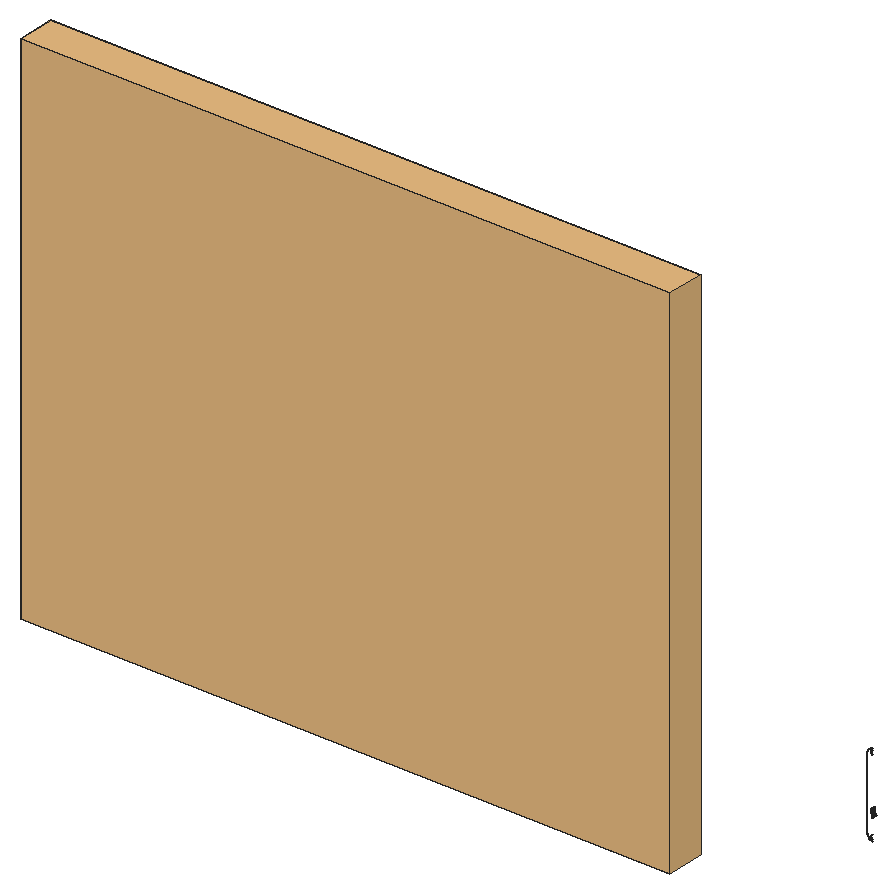
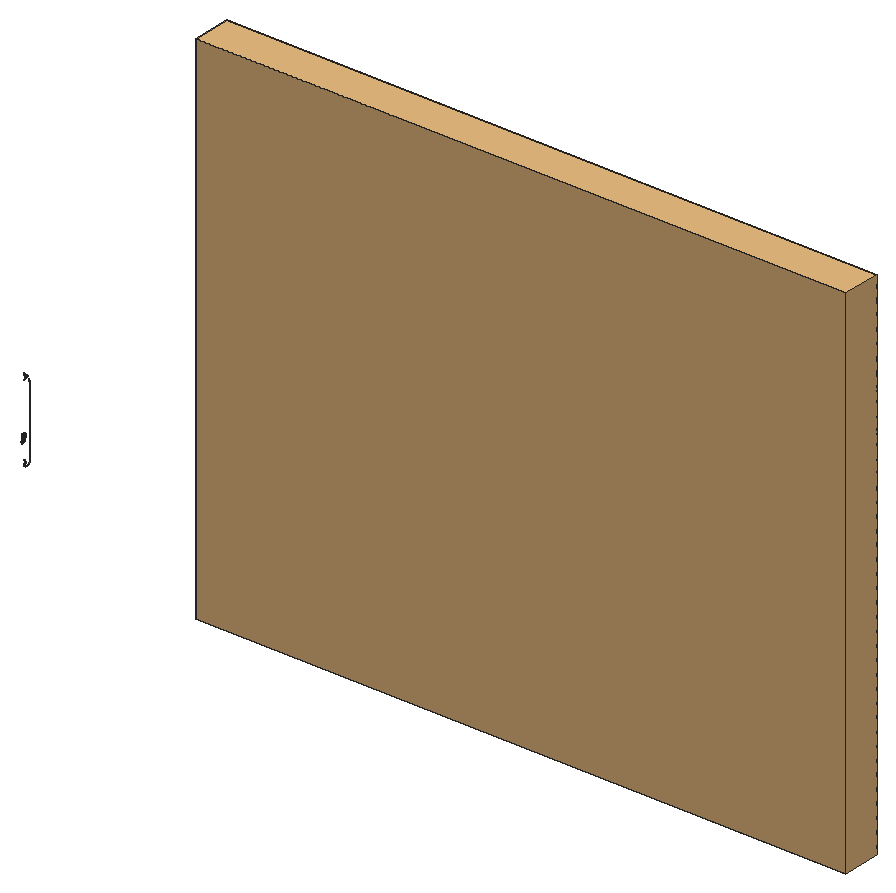
# SketchUp Ruby script. Lengths in inches.
U = 1.inch
M = Sketchup.active_model
def pt(a) = Geom::Point3d.new(a.map { |v| v * U })
def face(e, loops, mat)
  f = e.add_face(loops[0].map { |a| pt(a) })
  loops[1..].each { |l| e.add_face(l.map { |a| pt(a) }).erase! }
  f.material = f.back_material = mat if mat
  f
end
# faces: each face lists its corners as indices into pts; further lists are holes
def faces(e, pts, list, mat = nil) = list.each { |f| face(e, (f[0].is_a?(Array) ? f : [f]).map { |l| l.map { |i| pts[i] } }, mat) }
# xy, xz, yz: faces in a plane at the given z, y or x. An outline is a flat list of corners, or four numbers for a rectangle; further outlines are holes
def ring(l) = l.size == 4 ? [[l[0], l[1]], [l[2], l[1]], [l[2], l[3]], [l[0], l[3]]] : l.each_slice(2).to_a
def flat(e, list, mat, &to3) = list.each { |f| face(e, (f[0].is_a?(Array) ? f : [f]).map { |l| ring(l).map { |u, v| to3.(u, v) } }, mat) }
def xy(e, z, list, mat = nil) = flat(e, list, mat) { |x, y| [x, y, z] }
def xz(e, y, list, mat = nil) = flat(e, list, mat) { |x, z| [x, y, z] }
def yz(e, x, list, mat = nil) = flat(e, list, mat) { |y, z| [x, y, z] }
def lines(e, pts, list) = list.each { |a, b| e.add_line(pt(pts[a]), pt(pts[b])) }
# prism: a flat outline (further loops are holes) pulled along v
def prism(e, loops, v, mat = nil)
  f = face(e, loops, mat); d = Geom::Vector3d.new(v.map { |x| x * U })
  f.pushpull(f.normal.samedirection?(d) ? d.length : -d.length)
end
def box(e, o, s, mat = nil) = prism(e, [[o, [o[0] + s[0], o[1], o[2]], [o[0] + s[0], o[1] + s[1], o[2]], [o[0], o[1] + s[1], o[2]]]], [0, 0, s[2]], mat)
def at(x, y, z, deg = 0) = Geom::Transformation.translation(pt([x, y, z])) * Geom::Transformation.rotation(ORIGIN, Z_AXIS, deg.degrees)
def axes(o, x, y, z) = Geom::Transformation.new([*x, 0, *y, 0, *z, 0, *pt(o).to_a, 1])
def part(name) = M.definitions.add(name)
# library, detail: a bought-in or finely detailed component or shape, given as its bounding box
def library(name, o, s) = part(name).tap { |d| box(d.entities, o, s) }
def detail(e, o, s) = box(e.add_group.entities, o, s)
def put(e, d, t, mat = nil) = e.add_instance(d, t).tap { |i| i.material = mat if mat }
def group(e, t, mat = nil) = e.add_group.tap { |g| g.transformation = t; g.material = mat if mat }.entities
root = M.entities
M.materials.add("Material \#1").color = [140, 140, 140]
c1 = library("Multi-panel window",[0,0,0],[5.02,84.63,60])
xz(root,196.7,[[109.188,40.003,109.081,40.059,109.128,40.018],[109.188,40.003,109.128,40.018,109.157,40.007],[109.128,40.018,109.081,40.059,109.102,40.036],[109.295,40.059,108.945,40.647,109.046,40.46],[109.295,40.059,109.019,40.535,108.945,40.647],
  [109.295,40.059,109.053,40.498,109.019,40.535],[109.295,40.059,109.046,40.46,109.048,40.455],[109.295,40.059,109.048,40.455,109.05,40.45],[109.295,40.059,109.05,40.45,109.051,40.444],[109.081,40.059,109.051,40.438,109.054,40.118],
  [109.081,40.059,109.051,40.444,109.051,40.438],[109.081,40.059,109.295,40.059,109.051,40.444],[109.295,40.059,109.093,40.471,109.053,40.498],[109.081,40.059,109.054,40.118,109.065,40.087],[109.295,40.059,109.138,40.453,109.093,40.471],
  [109.054,40.118,109.051,40.438,109.051,40.152],[109.046,40.46,108.945,40.647,109.042,40.466],[109.042,40.466,108.945,40.647,109.039,40.47],[109.039,40.47,108.945,40.647,108.991,40.523],[109.039,40.47,108.991,40.523,109.034,40.475],
  [109.034,40.475,108.991,40.523,109.011,40.497],[108.991,40.523,108.945,40.647,108.961,40.581],[108.991,40.523,108.961,40.581,108.975,40.551],[109.019,40.535,108.993,40.579,108.945,40.647],[108.993,40.579,108.977,40.628,108.945,40.647],
  [108.961,40.581,108.945,40.647,108.951,40.613],[108.977,40.628,108.971,40.682,108.945,40.647],[108.945,40.647,108.949,40.743,108.943,40.682],[108.945,40.647,108.971,40.682,108.977,40.736],[108.945,40.647,108.977,40.736,108.996,40.849],
  [108.945,40.647,108.996,40.849,108.949,40.743],[108.977,40.736,108.993,40.786,108.996,40.849],[108.949,40.743,108.996,40.849,108.967,40.8],[108.993,40.786,109.019,40.829,108.996,40.849],[109.019,40.829,109.053,40.866,108.996,40.849],
  [108.996,40.849,109.053,40.866,109.093,40.894],[108.996,40.849,109.08,40.922,109.035,40.89],[108.996,40.849,109.093,40.894,109.188,40.949],[108.996,40.849,109.188,40.949,109.08,40.922],[109.093,40.894,109.138,40.912,109.188,40.949],
  [109.138,40.912,109.188,40.918,109.188,40.949],[109.08,40.922,109.188,40.949,109.132,40.942]],"Material \#1")
xz(root,196.734,[[109.188,37.641,109.188,37.652,109.074,37.652],[109.074,37.652,109.076,37.663,108.968,37.684],[109.074,37.652,109.188,37.652,109.076,37.663],[109.076,37.663,108.972,37.695,108.968,37.684],[108.968,37.684,108.972,37.695,108.869,37.734],
  [108.972,37.695,108.875,37.745,108.869,37.734],[108.869,37.734,108.875,37.745,108.781,37.802],[108.875,37.745,108.788,37.811,108.781,37.802],[108.781,37.802,108.788,37.811,108.705,37.885],[108.788,37.811,108.713,37.893,108.705,37.885],
  [109.188,37.824,109.188,37.836,109.151,37.828],[109.151,37.828,109.152,37.84,109.115,37.839],[109.151,37.828,109.188,37.836,109.152,37.84],[109.115,37.839,109.119,37.85,109.082,37.855],[109.115,37.839,109.152,37.84,109.119,37.85],
  [109.119,37.85,109.088,37.866,109.082,37.855],[109.082,37.855,109.088,37.866,109.053,37.878],[109.088,37.866,109.06,37.887,109.053,37.878],[109.053,37.878,109.06,37.887,109.028,37.905],[108.705,37.885,108.713,37.893,108.646,37.975],
  [109.06,37.887,109.036,37.913,109.028,37.905],[108.713,37.893,108.655,37.981,108.646,37.975],[109.028,37.905,109.036,37.913,109.007,37.937],[109.036,37.913,109.016,37.943,109.007,37.937],[109.007,37.937,109.016,37.943,108.991,37.973],
  [109.016,37.943,109.002,37.977,108.991,37.973],[108.991,37.973,109.002,37.977,108.982,38.011],[108.646,37.975,108.655,37.981,108.596,38.088],[109.002,37.977,108.992,38.014,108.982,38.011],[108.655,37.981,108.606,38.092,108.596,38.088],
  [108.982,38.011,108.992,38.014,108.978,38.048],[108.992,38.014,108.989,38.048,108.978,38.048],[108.978,38.048,108.989,38.048,108.982,38.093],[108.989,38.048,108.992,38.091,108.982,38.093],[108.596,38.088,108.606,38.092,108.567,38.204],
  [108.992,38.091,108.991,38.132,108.982,38.093],[108.992,38.091,109.002,38.128,108.991,38.132],[108.606,38.092,108.577,38.206,108.567,38.204],[109.002,38.128,109.007,38.167,108.991,38.132],[109.002,38.128,109.016,38.161,109.007,38.167],
  [109.016,38.161,109.028,38.199,109.007,38.167],[109.016,38.161,109.036,38.192,109.028,38.199],[109.036,38.192,109.053,38.227,109.028,38.199],[109.036,38.192,109.06,38.218,109.053,38.227],[108.567,38.204,108.577,38.206,108.556,38.331],
  [108.577,38.206,108.567,38.332,108.556,38.331],[109.06,38.218,109.082,38.249,109.053,38.227],[109.06,38.218,109.088,38.239,109.082,38.249],[109.088,38.239,109.115,38.266,109.082,38.249],[109.088,38.239,109.119,38.255,109.115,38.266],
  [109.119,38.255,109.151,38.277,109.115,38.266],[109.119,38.255,109.152,38.265,109.151,38.277],[109.152,38.265,109.188,38.28,109.151,38.277],[109.152,38.265,109.188,38.269,109.188,38.28],[108.556,38.331,108.567,38.332,108.556,46.173],
  [108.567,38.332,108.567,46.173,108.556,46.173],[108.556,46.173,108.567,46.173,108.567,46.301],[108.567,46.173,108.577,46.299,108.567,46.301],[109.188,46.224,109.188,46.236,109.151,46.228],[109.151,46.228,109.152,46.24,109.115,46.239],
  [109.151,46.228,109.188,46.236,109.152,46.24],[109.115,46.239,109.119,46.25,109.082,46.255],[109.115,46.239,109.152,46.24,109.119,46.25],[109.119,46.25,109.088,46.266,109.082,46.255],[109.082,46.255,109.088,46.266,109.053,46.278],
  [109.088,46.266,109.06,46.287,109.053,46.278],[109.053,46.278,109.06,46.287,109.028,46.305],[109.06,46.287,109.036,46.313,109.028,46.305],[108.577,46.299,108.596,46.417,108.567,46.301],[108.577,46.299,108.606,46.413,108.596,46.417],
  [109.028,46.305,109.036,46.313,109.007,46.337],[109.036,46.313,109.016,46.343,109.007,46.337],[109.007,46.337,109.016,46.343,108.991,46.373],[109.016,46.343,109.002,46.377,108.991,46.373],[108.991,46.373,109.002,46.377,108.982,46.412],
  [109.002,46.377,108.992,46.414,108.982,46.412],[108.982,46.412,108.992,46.414,108.978,46.463],[108.606,46.413,108.643,46.524,108.596,46.417],[108.606,46.413,108.652,46.518,108.643,46.524],[108.992,46.414,108.989,46.463,108.978,46.463],
  [108.978,46.463,108.989,46.463,108.982,46.493],[108.989,46.463,108.992,46.491,108.982,46.493],[108.992,46.491,108.991,46.532,108.982,46.493],[108.992,46.491,109.002,46.528,108.991,46.532],[108.652,46.518,108.708,46.623,108.643,46.524],
  [108.652,46.518,108.716,46.615,108.708,46.623],[109.002,46.528,109.007,46.567,108.991,46.532],[109.002,46.528,109.016,46.561,109.007,46.567],[109.016,46.561,109.028,46.599,109.007,46.567],[109.016,46.561,109.036,46.592,109.028,46.599],
  [109.036,46.592,109.053,46.627,109.028,46.599],[109.036,46.592,109.06,46.618,109.053,46.627],[108.716,46.615,108.781,46.703,108.708,46.623],[108.716,46.615,108.788,46.693,108.781,46.703],[109.06,46.618,109.082,46.649,109.053,46.627],
  [109.06,46.618,109.088,46.639,109.082,46.649],[109.088,46.639,109.115,46.666,109.082,46.649],[109.088,46.639,109.119,46.655,109.115,46.666],[109.119,46.655,109.151,46.677,109.115,46.666],[109.119,46.655,109.152,46.665,109.151,46.677],
  [109.152,46.665,109.188,46.68,109.151,46.677],[108.788,46.693,108.869,46.77,108.781,46.703],[108.788,46.693,108.875,46.76,108.869,46.77],[108.875,46.76,108.968,46.821,108.869,46.77],[108.875,46.76,108.972,46.81,108.968,46.821],
  [108.972,46.81,109.074,46.853,108.968,46.821],[108.972,46.81,109.076,46.841,109.074,46.853],[109.076,46.841,109.188,46.864,109.074,46.853],[109.076,46.841,109.188,46.852,109.188,46.864]],"Material \#1")
xz(root,197.036,[[109.188,40.003,109.157,40.007,109.128,40.018],[109.128,40.018,109.051,40.438,109.322,40.118],[109.128,40.018,109.054,40.118,109.051,40.438],[109.128,40.018,109.081,40.059,109.054,40.118],[109.128,40.018,109.102,40.036,109.081,40.059],
  [109.081,40.059,109.065,40.087,109.054,40.118],[109.322,40.118,109.048,40.455,109.046,40.46],[109.322,40.118,109.05,40.45,109.048,40.455],[109.322,40.118,109.051,40.444,109.05,40.45],[109.054,40.118,109.051,40.152,109.051,40.438],
  [109.322,40.118,109.051,40.438,109.051,40.444],[109.325,40.152,109.019,40.535,109.053,40.498],[109.325,40.152,109.046,40.46,109.019,40.535],[109.325,40.152,109.053,40.498,109.093,40.471],[109.046,40.46,108.945,40.647,108.993,40.579],
  [109.046,40.46,109.042,40.466,108.945,40.647],[109.046,40.46,108.993,40.579,109.019,40.535],[109.042,40.466,109.039,40.47,108.945,40.647],[109.039,40.47,108.991,40.523,108.945,40.647],[109.039,40.47,109.034,40.475,108.991,40.523],
  [109.034,40.475,109.011,40.497,108.991,40.523],[108.991,40.523,108.961,40.581,108.945,40.647],[108.991,40.523,108.975,40.551,108.961,40.581],[108.993,40.579,108.945,40.647,108.977,40.628],[108.961,40.581,108.951,40.613,108.945,40.647],
  [108.977,40.628,108.945,40.647,108.971,40.682],[108.945,40.647,108.943,40.682,108.949,40.743],[108.945,40.647,108.949,40.743,108.996,40.849],[108.945,40.647,108.977,40.736,108.971,40.682],[108.945,40.647,108.993,40.786,108.977,40.736],
  [108.945,40.647,108.996,40.849,108.993,40.786],[108.949,40.743,108.967,40.8,108.996,40.849],[108.993,40.786,108.996,40.849,109.019,40.829],[109.019,40.829,108.996,40.849,109.053,40.866],[108.996,40.849,109.035,40.89,109.08,40.922],
  [108.996,40.849,109.08,40.922,109.188,40.949],[108.996,40.849,109.093,40.894,109.053,40.866],[108.996,40.849,109.188,40.949,109.093,40.894],[109.093,40.894,109.188,40.949,109.138,40.912],[109.08,40.922,109.132,40.942,109.188,40.949]],"Material \#1")
yz(root,109.162,[[197.002,40.788,197.002,40.839,196.69,40.839]],"Material \#1")
yz(root,109.167,[[197.002,40.582,197.002,40.612,196.69,40.612]],"Material \#1")
p = [[109.165,196.69,40.553],[109.167,197.002,40.549],[109.162,197.002,40.557],[109.167,197.002,40.639],[109.159,197.002,40.661],[109.159,196.69,40.672],
  [109.165,196.69,40.578],[109.165,196.69,40.553],[109.162,197.002,40.557],[109.162,197.002,40.574],[109.159,196.69,40.672],[109.163,196.69,40.65],
  [109.167,197.002,40.639],[109.165,196.69,40.578],[109.162,197.002,40.574],[109.167,197.002,40.582],[109.163,196.69,40.65],[109.167,196.69,40.612],
  [109.167,197.002,40.612],[109.167,197.002,40.612],[109.167,197.002,40.639],[109.163,196.69,40.65],[109.167,196.69,40.612],[109.165,196.69,40.578],
  [109.167,197.002,40.582],[109.159,197.002,40.661],[109.159,197.002,40.684],[109.163,196.69,40.695],[109.163,196.69,40.695],[109.159,196.69,40.672],
  [109.159,197.002,40.661],[109.165,196.69,40.714],[109.163,196.69,40.695],[109.159,197.002,40.684],[109.162,197.002,40.721],[109.162,197.002,40.773],
  [109.165,196.69,40.777],[109.165,196.69,40.777],[109.162,196.69,40.725],[109.162,197.002,40.721],[109.159,197.002,40.684],[109.167,197.002,40.706],
  [109.165,196.69,40.714],[109.167,197.002,40.706],[109.162,197.002,40.721],[109.162,196.69,40.725],[109.162,196.69,40.725],[109.165,196.69,40.714],
  [109.167,197.002,40.706],[109.162,196.69,40.839],[109.165,196.69,40.777],[109.162,197.002,40.788]]
faces(root,p,[[0,1,2],[3,4,5],[6,7,8],[8,9,6],[10,11,12],[13,14,15],[16,17,18],[19,20,21],
  [22,23,24],[25,26,27],[28,29,30],[31,32,33],[34,35,36],[37,38,39],[40,41,42],[43,44,45],
  [46,47,48],[49,50,51]],"Material \#1")
put(root,c1,axes([17.84,197.02,29.375],[0,-0.84,0],[0.85075,0,0],[0,0,0.96039]))
